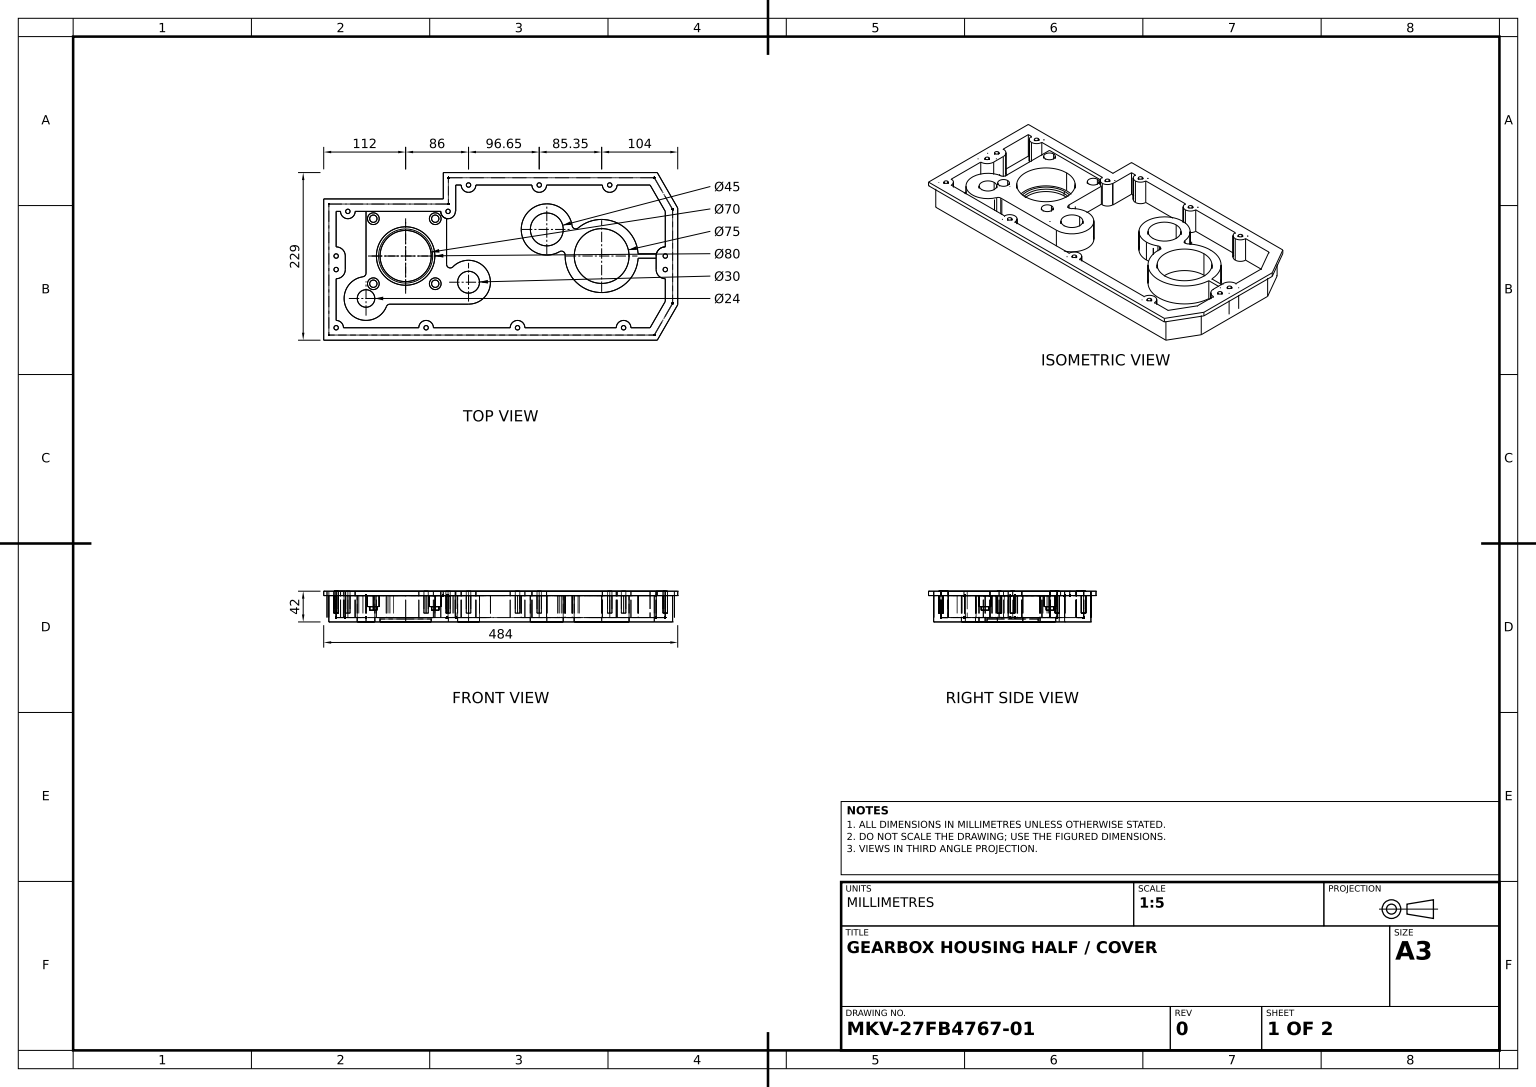
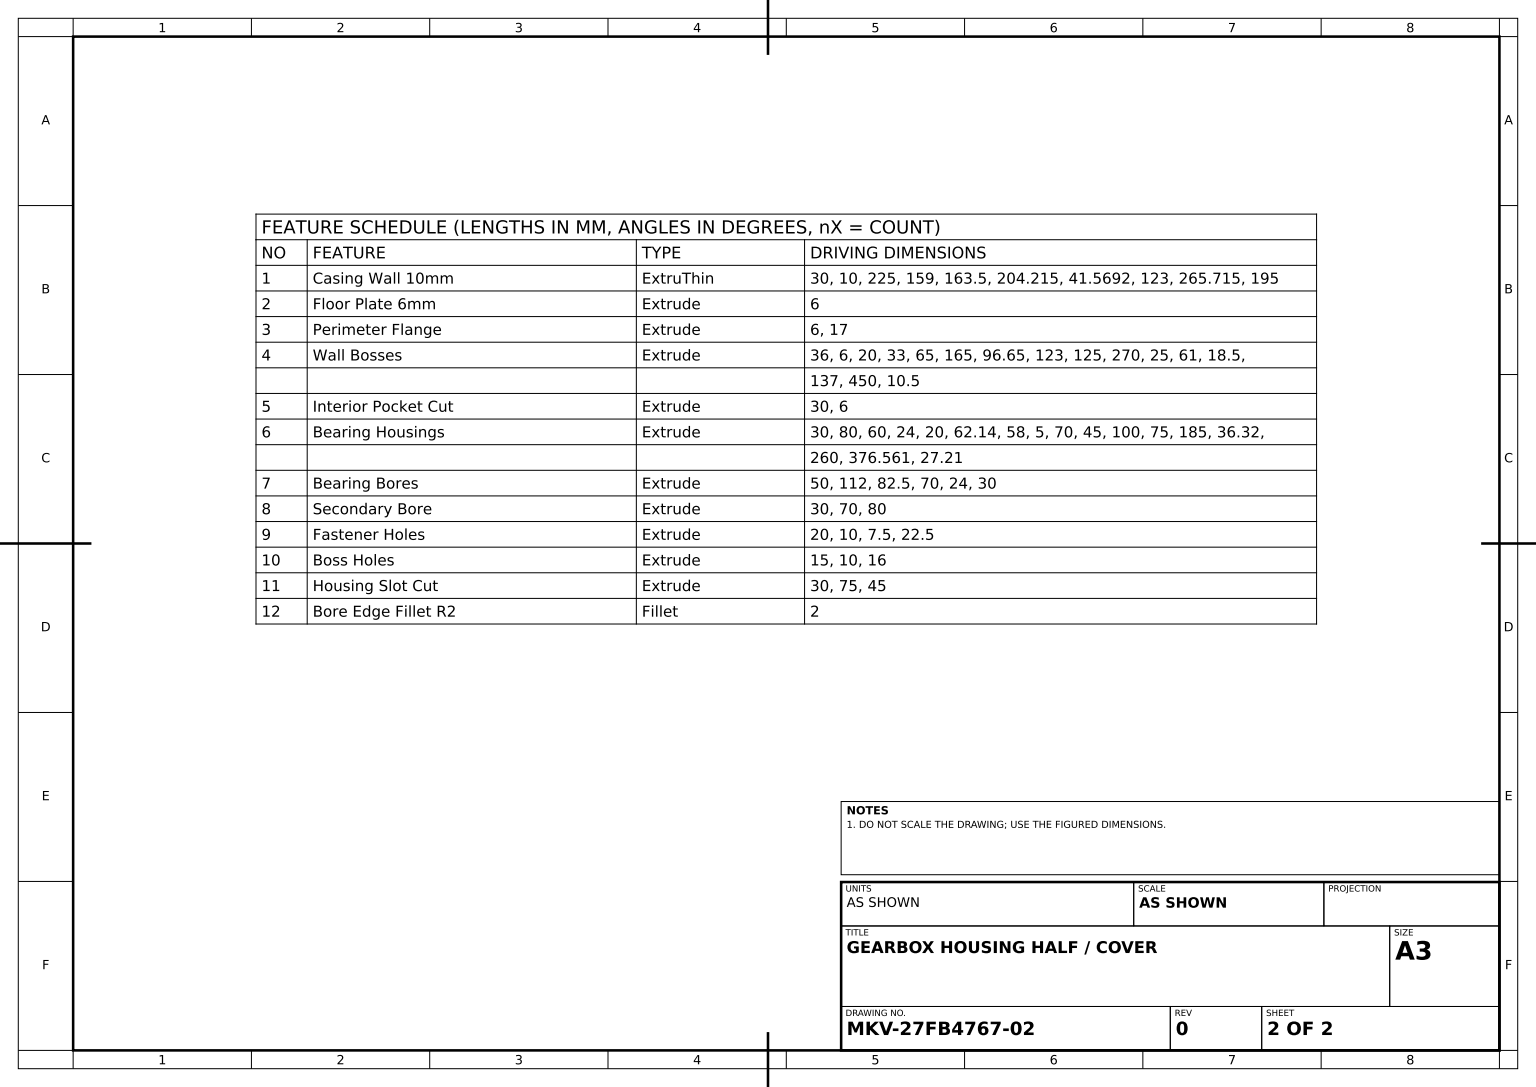
solid
v1 (225,36,-159)
v2 (204.21539,36,-195)
e1 v1 v2 LINE
v3 (204.21539,0,-195)
e2 v2 v3 LINE
v4 (225,0,-159)
e3 v4 v3 LINE
e4 v1 v4 LINE
face PLANE(AX(P(225,30,-159),D(-0.866025404,0,0.5),D(0.5,0,0.866025404))) [e1 e2 -e3 -e4]
v5 (-209,6,-162)
v6 (-209,36,-162)
e5 v5 v6 LINE
v7 (-209,6,-156)
e6 v7 v5 CIRCLE(AX(P(-209,6,-159),D(0,1,0),D(0,0,1)),3)
v8 (-209,36,-156)
e7 v7 v8 LINE
e8 v8 v6 CIRCLE(AX(P(-209,36,-159),D(0,1,0),D(0,0,1)),3)
face CYL(AX(P(-209,6,-159),D(0,1,0),D(0,0,1)),3) rev [-e5 -e6 e7 e8]
e9 v5 v7 CIRCLE(AX(P(-209,6,-159),D(0,1,0),D(0,0,1)),3)
face PLANE(AX(P(-209,6,-159),D(0,1,0),D(0,0,1))) [e9 e6]
v9 (-34,0,-195)
v10 (-34,36,-195)
e10 v9 v10 LINE
v11 (-44,36,-185)
e11 v11 v10 CIRCLE(AX(P(-44,36,-195),D(0,1,0),D(0,0,1)),10)
v12 (-44,0,-185)
e12 v12 v11 LINE
e13 v12 v9 CIRCLE(AX(P(-44,0,-195),D(0,1,0),D(0,0,1)),10)
face CYL(AX(P(-44,0,-195),D(0,1,0),D(0,0,1)),10) [e10 -e11 -e12 e13]
v13 (-89.5,30,-157)
v14 (-89.5,30,-141)
e14 v13 v14 CIRCLE(AX(P(-89.5,30,-149),D(0,1,0),D(0,0,1)),8)
v15 (-89.5,15,-141)
e15 v15 v14 LINE
v16 (-89.5,15,-157)
e16 v16 v15 CIRCLE(AX(P(-89.5,15,-149),D(0,1,0),D(0,0,1)),8)
e17 v16 v13 LINE
face CYL(AX(P(-89.5,15,-149),D(0,1,0),D(0,0,1)),8) rev [e14 -e15 -e16 e17]
v17 (242,36,-31.444864)
v18 (242,30,-31.444864)
e18 v17 v18 LINE
v19 (214.030345,36,17)
e19 v19 v17 LINE
v20 (214.030345,30,17)
e20 v19 v20 LINE
e21 v20 v18 LINE
face PLANE(AX(P(242,36,-31.444864),D(-0.866025404,0,-0.5),D(-0.5,0,0.866025404))) rev [-e18 -e19 e20 e21]
v21 (-44,30,-47.21)
v22 (-44,-6,-47.21)
e22 v21 v22 LINE
v23 (-44,-6,-77.21)
e23 v22 v23 CIRCLE(AX(P(-44,-6,-62.21),D(0,-1,0),D(0,0,-1)),15)
v24 (-44,30,-77.21)
e24 v24 v23 LINE
e25 v24 v21 CIRCLE(AX(P(-44,30,-62.21),D(0,1,0),D(0,0,1)),15)
face CYL(AX(P(-44,30,-62.21),D(0,-1,0),D(0,0,-1)),15) rev [e22 e23 -e24 e25]
v25 (159.030345,0,-195)
e26 v3 v25 LINE
v26 (159.030345,36,-195)
e27 v2 v26 LINE
e28 v25 v26 LINE
face PLANE(AX(P(-61.5,30,-195),D(0,0,1),D(1,0,0))) [-e26 -e2 e27 -e28]
v27 (-72,6,-162)
v28 (-72,36,-162)
e29 v27 v28 LINE
v29 (-72,36,-156)
e30 v28 v29 CIRCLE(AX(P(-72,36,-159),D(0,1,0),D(0,0,1)),3)
v30 (-72,6,-156)
e31 v30 v29 LINE
e32 v27 v30 CIRCLE(AX(P(-72,6,-159),D(0,1,0),D(0,0,1)),3)
face CYL(AX(P(-72,6,-159),D(0,1,0),D(0,0,1)),3) rev [e29 e30 -e31 -e32]
v31 (-215,0,0)
v32 (-215,36,0)
e33 v31 v32 LINE
v33 (-112,36,0)
e34 v32 v33 LINE
v34 (-112,0,0)
e35 v34 v33 LINE
e36 v31 v34 LINE
face PLANE(AX(P(-225,30,0),D(0,0,-1),D(-1,0,0))) [e33 e34 -e35 -e36]
v35 (139.030345,0,-195)
v36 (149.030345,0,-185)
e37 v35 v36 CIRCLE(AX(P(149.030345,0,-195),D(0,1,0),D(0,0,1)),10)
v37 (149.030345,36,-185)
e38 v36 v37 LINE
v38 (139.030345,36,-195)
e39 v38 v37 CIRCLE(AX(P(149.030345,36,-195),D(0,1,0),D(0,0,1)),10)
e40 v35 v38 LINE
face CYL(AX(P(149.030345,0,-195),D(0,1,0),D(0,0,1)),10) [e37 e38 -e39 -e40]
v39 (52.65,36,-192)
v40 (52.65,36,-198)
e41 v39 v40 CIRCLE(AX(P(52.65,36,-195),D(0,1,0),D(0,0,1)),3)
v41 (52.65,6,-198)
e42 v41 v40 LINE
v42 (52.65,6,-192)
e43 v42 v41 CIRCLE(AX(P(52.65,6,-195),D(0,1,0),D(0,0,1)),3)
e44 v42 v39 LINE
face CYL(AX(P(52.65,6,-195),D(0,1,0),D(0,0,1)),3) rev [e41 -e42 -e43 e44]
v43 (-225,0,-67)
v44 (-225,0,-10)
e45 v43 v44 LINE
v45 (-225,36,-67)
e46 v43 v45 LINE
v46 (-225,36,-10)
e47 v45 v46 LINE
e48 v44 v46 LINE
face PLANE(AX(P(-225,30,0),D(1,0,0),D(0,0,-1))) [-e45 e46 e47 -e48]
v47 (42.65,36,-195)
e49 v47 v10 LINE
v48 (42.65,0,-195)
e50 v48 v9 LINE
e51 v48 v47 LINE
face PLANE(AX(P(-61.5,30,-195),D(0,0,1),D(1,0,0))) [e49 -e10 -e50 e51]
v49 (63,30,-111.82)
v50 (63,-6,-111.82)
e52 v49 v50 LINE
v51 (63,30,-156.82)
e53 v49 v51 CIRCLE(AX(P(63,30,-134.32),D(0,1,0),D(0,0,1)),22.5)
v52 (63,-6,-156.82)
e54 v51 v52 LINE
e55 v52 v50 CIRCLE(AX(P(63,-6,-134.32),D(0,-1,0),D(0,0,-1)),22.5)
face CYL(AX(P(63,30,-134.32),D(0,-1,0),D(0,0,-1)),22.5) rev [-e52 e53 e54 e55]
e56 v30 v27 CIRCLE(AX(P(-72,6,-159),D(0,1,0),D(0,0,1)),3)
face PLANE(AX(P(-72,6,-159),D(0,1,0),D(0,0,1))) [e32 e56]
v53 (-102,36,-3)
v54 (-102,36,3)
e57 v53 v54 CIRCLE(AX(P(-102,36,0),D(0,1,0),D(0,0,1)),3)
v55 (-102,6,3)
e58 v55 v54 LINE
v56 (-102,6,-3)
e59 v56 v55 CIRCLE(AX(P(-102,6,0),D(0,1,0),D(0,0,1)),3)
e60 v56 v53 LINE
face CYL(AX(P(-102,6,0),D(0,1,0),D(0,0,1)),3) rev [e57 -e58 -e59 e60]
v57 (209.988893,30,10)
v58 (209.988893,-6,10)
e61 v57 v58 LINE
v59 (-235,30,10)
e62 v59 v57 LINE
v60 (-235,-6,10)
e63 v59 v60 LINE
e64 v58 v60 LINE
face PLANE(AX(P(0,30,10),D(0,0,-1),D(-1,0,0))) rev [-e61 -e62 e63 -e64]
v61 (225,6,-76.5)
v62 (225,6,-82.5)
e65 v61 v62 CIRCLE(AX(P(225,6,-79.5),D(0,1,0),D(0,0,1)),3)
v63 (225,36,-76.5)
e66 v61 v63 LINE
v64 (225,36,-82.5)
e67 v63 v64 CIRCLE(AX(P(225,36,-79.5),D(0,1,0),D(0,0,1)),3)
e68 v62 v64 LINE
face CYL(AX(P(225,6,-79.5),D(0,1,0),D(0,0,1)),3) rev [-e65 e66 e67 -e68]
v65 (80.522834,30,-104.022305)
v66 (80.522834,0,-104.022305)
e69 v65 v66 LINE
v67 (83.026096,0,-104.694063)
e70 v67 v66 CIRCLE(AX(P(83.026096,0,-99.694063),D(0,1,0),D(0,0,1)),5)
v68 (83.026096,30,-104.694063)
e71 v68 v67 LINE
e72 v68 v65 CIRCLE(AX(P(83.026096,30,-99.694063),D(0,1,0),D(0,0,1)),5)
face CYL(AX(P(83.026096,30,-99.694063),D(0,-1,0),D(0,0,-1)),5) rev [e69 -e70 -e71 e72]
v69 (-130,-6,-63)
v70 (-130,-6,-133)
e73 v69 v70 CIRCLE(AX(P(-130,-6,-98),D(0,-1,0),D(0,0,-1)),35)
e74 v70 v69 CIRCLE(AX(P(-130,-6,-98),D(0,-1,0),D(0,0,-1)),35)
v71 (235,-6,-33.320508)
e75 v71 v58 LINE
v72 (-235,-6,-169)
e76 v60 v72 LINE
v73 (-71.5,-6,-169)
e77 v72 v73 LINE
v74 (-71.5,-6,-205)
e78 v73 v74 LINE
v75 (209.988893,-6,-205)
e79 v74 v75 LINE
v76 (235,-6,-161.679492)
e80 v75 v76 LINE
e81 v76 v71 LINE
e82 v23 v22 CIRCLE(AX(P(-44,-6,-62.21),D(0,-1,0),D(0,0,-1)),15)
v77 (-184.14,-6,-28)
v78 (-184.14,-6,-52)
e83 v77 v78 CIRCLE(AX(P(-184.14,-6,-40),D(0,-1,0),D(0,0,-1)),12)
e84 v78 v77 CIRCLE(AX(P(-184.14,-6,-40),D(0,-1,0),D(0,0,-1)),12)
v79 (138,-6,-135.5)
v80 (138,-6,-60.5)
e85 v79 v80 CIRCLE(AX(P(138,-6,-98),D(0,-1,0),D(0,0,-1)),37.5)
e86 v80 v79 CIRCLE(AX(P(138,-6,-98),D(0,-1,0),D(0,0,-1)),37.5)
e87 v50 v52 CIRCLE(AX(P(63,-6,-134.32),D(0,-1,0),D(0,0,-1)),22.5)
face PLANE(AX(P(0,-6,0),D(0,-1,0),D(0,0,-1))) [-e73 -e74] [e75 e64 e76 e77 e78 e79 e80 e81] [-e23 -e82] [-e83 -e84] [-e85 -e86] [-e55 -e87]
v81 (187.909919,30,-101)
v82 (212.865339,30,-101)
e88 v81 v82 LINE
v83 (212.865339,0,-101)
e89 v82 v83 LINE
v84 (187.909919,0,-101)
e90 v84 v83 LINE
e91 v81 v84 LINE
face PLANE(AX(P(0,30,-101),D(0,0,-1),D(-1,0,0))) [e88 e89 -e90 -e91]
v85 (242,36,-163.555136)
v86 (242,30,-163.555136)
e92 v85 v86 LINE
e93 v17 v85 LINE
e94 v18 v86 LINE
face PLANE(AX(P(242,36,-163.555136),D(-1,0,0),D(0,0,1))) rev [-e92 -e93 e18 e94]
v87 (-62,0,-159)
v88 (-62,36,-159)
e95 v87 v88 LINE
v89 (-72,36,-149)
e96 v89 v88 CIRCLE(AX(P(-72,36,-159),D(0,1,0),D(0,0,1)),10)
v90 (-72,0,-149)
e97 v90 v89 LINE
e98 v90 v87 CIRCLE(AX(P(-72,0,-159),D(0,1,0),D(0,0,1)),10)
face CYL(AX(P(-72,0,-159),D(0,1,0),D(0,0,1)),10) [e95 -e96 -e97 e98]
v91 (-225,36,-101)
v92 (-225,36,-95)
e99 v91 v92 CIRCLE(AX(P(-225,36,-98),D(0,1,0),D(0,0,1)),3)
v93 (-225,6,-95)
e100 v93 v92 LINE
v94 (-225,6,-101)
e101 v94 v93 CIRCLE(AX(P(-225,6,-98),D(0,1,0),D(0,0,1)),3)
e102 v94 v91 LINE
face CYL(AX(P(-225,6,-98),D(0,1,0),D(0,0,1)),3) rev [e99 -e100 -e101 e102]
v95 (-209,0,-149)
v96 (-209,36,-149)
e103 v95 v96 LINE
v97 (-219,36,-159)
e104 v97 v96 CIRCLE(AX(P(-209,36,-159),D(0,1,0),D(0,0,1)),10)
v98 (-219,0,-159)
e105 v98 v97 LINE
e106 v98 v95 CIRCLE(AX(P(-209,0,-159),D(0,1,0),D(0,0,1)),10)
face CYL(AX(P(-209,0,-159),D(0,1,0),D(0,0,1)),10) [e103 -e104 -e105 e106]
v99 (23,6,-3)
v100 (23,36,-3)
e107 v99 v100 LINE
v101 (23,36,3)
e108 v100 v101 CIRCLE(AX(P(23,36,0),D(0,1,0),D(0,0,1)),3)
v102 (23,6,3)
e109 v102 v101 LINE
e110 v99 v102 CIRCLE(AX(P(23,6,0),D(0,1,0),D(0,0,1)),3)
face CYL(AX(P(23,6,0),D(0,1,0),D(0,0,1)),3) rev [e107 e108 -e109 -e110]
v103 (-174.14,10,-144)
v104 (-174.14,15,-144)
e111 v103 v104 LINE
v105 (-174.14,10,-154)
e112 v105 v103 CIRCLE(AX(P(-174.14,10,-149),D(0,1,0),D(0,0,1)),5)
v106 (-174.14,15,-154)
e113 v105 v106 LINE
e114 v106 v104 CIRCLE(AX(P(-174.14,15,-149),D(0,1,0),D(0,0,1)),5)
face CYL(AX(P(-174.14,10,-149),D(0,1,0),D(0,0,1)),5) rev [-e111 -e112 e113 e114]
v107 (-225,36,-3)
v108 (-225,36,3)
e115 v107 v108 CIRCLE(AX(P(-225,36,0),D(0,1,0),D(0,0,1)),3)
v109 (-225,6,3)
e116 v109 v108 LINE
v110 (-225,6,-3)
e117 v110 v109 CIRCLE(AX(P(-225,6,0),D(0,1,0),D(0,0,1)),3)
e118 v110 v107 LINE
face CYL(AX(P(-225,6,0),D(0,1,0),D(0,0,1)),3) rev [e115 -e116 -e117 e118]
v111 (-156.214818,30,-29.037143)
v112 (-156.214818,0,-29.037143)
e119 v111 v112 LINE
v113 (-188.425714,30,-69.6923)
e120 v113 v111 CIRCLE(AX(P(-184.14,30,-40),D(0,1,0),D(0,0,1)),30)
v114 (-188.425714,0,-69.6923)
e121 v113 v114 LINE
e122 v114 v112 CIRCLE(AX(P(-184.14,0,-40),D(0,1,0),D(0,0,1)),30)
face CYL(AX(P(-184.14,30,-40),D(0,-1,0),D(0,0,-1)),30) [-e119 -e120 e121 e122]
v115 (-130,0,-58)
v116 (-130,0,-138)
e123 v115 v116 CIRCLE(AX(P(-130,0,-98),D(0,1,0),D(0,0,1)),40)
e124 v116 v115 CIRCLE(AX(P(-130,0,-98),D(0,1,0),D(0,0,1)),40)
v117 (-130,0,-61)
v118 (-130,0,-135)
e125 v117 v118 CIRCLE(AX(P(-130,0,-98),D(0,-1,0),D(0,0,1)),37)
e126 v118 v117 CIRCLE(AX(P(-130,0,-98),D(0,-1,0),D(0,0,1)),37)
face PLANE(AX(P(-130,0,-98),D(0,1,0),D(0,0,1))) [e123 e124] [e125 e126]
v119 (88.023723,30,-99.540058)
v120 (187.909919,30,-95)
e127 v119 v120 CIRCLE(AX(P(138,30,-98),D(0,1,0),D(0,0,1)),50)
v121 (88.023723,0,-99.540058)
e128 v119 v121 LINE
v122 (187.909919,0,-95)
e129 v121 v122 CIRCLE(AX(P(138,0,-98),D(0,1,0),D(0,0,1)),50)
e130 v120 v122 LINE
face CYL(AX(P(138,30,-98),D(0,-1,0),D(0,0,-1)),50) [-e127 e128 e129 -e130]
v123 (-89.5,15,-68.155644)
v124 (-89.5,15,-52.155644)
e131 v123 v124 CIRCLE(AX(P(-89.5,15,-60.155644),D(0,1,0),D(0,0,1)),8)
e132 v124 v123 CIRCLE(AX(P(-89.5,15,-60.155644),D(0,1,0),D(0,0,1)),8)
v125 (-89.5,15,-55.155644)
v126 (-89.5,15,-65.155644)
e133 v125 v126 CIRCLE(AX(P(-89.5,15,-60.155644),D(0,1,0),D(0,0,1)),5)
e134 v126 v125 CIRCLE(AX(P(-89.5,15,-60.155644),D(0,1,0),D(0,0,1)),5)
face PLANE(AX(P(-89.5,15,-60.155644),D(0,1,0),D(0,0,1))) [e131 e132] [-e133 -e134]
v127 (225,6,-101)
v128 (225,36,-101)
e135 v127 v128 LINE
v129 (225,6,-95)
e136 v129 v127 CIRCLE(AX(P(225,6,-98),D(0,1,0),D(0,0,1)),3)
v130 (225,36,-95)
e137 v129 v130 LINE
e138 v130 v128 CIRCLE(AX(P(225,36,-98),D(0,1,0),D(0,0,1)),3)
face CYL(AX(P(225,6,-98),D(0,1,0),D(0,0,1)),3) rev [-e135 -e136 e137 e138]
v131 (212.5,30,-98)
v132 (212.5,36,-98)
e139 v131 v132 LINE
v133 (212.5,30,-95)
e140 v133 v131 LINE
v134 (212.5,0,-95)
e141 v133 v134 LINE
v135 (212.5,0,-79.5)
e142 v134 v135 LINE
v136 (212.5,36,-79.5)
e143 v135 v136 LINE
e144 v132 v136 LINE
face PLANE(AX(P(212.5,0,0),D(-1,0,0),D(0,0,1))) [-e139 -e140 e141 e142 e143 -e144]
v137 (-225,36,-159)
e145 v97 v137 LINE
v138 (-225,0,-159)
e146 v137 v138 LINE
e147 v98 v138 LINE
face PLANE(AX(P(-225,30,-159),D(0,0,1),D(1,0,0))) [e105 e145 e146 -e147]
v139 (-225,6,-82.5)
v140 (-225,36,-82.5)
e148 v139 v140 LINE
v141 (-225,6,-76.5)
e149 v141 v139 CIRCLE(AX(P(-225,6,-79.5),D(0,1,0),D(0,0,1)),3)
v142 (-225,36,-76.5)
e150 v141 v142 LINE
e151 v142 v140 CIRCLE(AX(P(-225,36,-79.5),D(0,1,0),D(0,0,1)),3)
face CYL(AX(P(-225,6,-79.5),D(0,1,0),D(0,0,1)),3) rev [-e148 -e149 e150 e151]
v143 (-89.5,15,-154)
v144 (-89.5,15,-144)
e152 v143 v144 CIRCLE(AX(P(-89.5,15,-149),D(0,1,0),D(0,0,1)),5)
v145 (-89.5,10,-144)
e153 v145 v144 LINE
v146 (-89.5,10,-154)
e154 v146 v145 CIRCLE(AX(P(-89.5,10,-149),D(0,1,0),D(0,0,1)),5)
e155 v146 v143 LINE
face CYL(AX(P(-89.5,10,-149),D(0,1,0),D(0,0,1)),5) rev [e152 -e153 -e154 e155]
v147 (-44,30,-32.21)
v148 (-151.560622,30,-32.21)
e156 v147 v148 LINE
v149 (-151.560622,0,-32.21)
e157 v148 v149 LINE
v150 (-44,0,-32.21)
e158 v150 v149 LINE
e159 v147 v150 LINE
face PLANE(AX(P(0,30,-32.21),D(0,0,1),D(1,0,0))) [e156 e157 -e158 -e159]
v151 (-89.5,30,-68.155644)
e160 v123 v151 LINE
v152 (-89.5,30,-52.155644)
e161 v151 v152 CIRCLE(AX(P(-89.5,30,-60.155644),D(0,1,0),D(0,0,1)),8)
e162 v124 v152 LINE
face CYL(AX(P(-89.5,15,-60.155644),D(0,1,0),D(0,0,1)),8) rev [e160 e161 -e162 -e131]
v153 (62.65,36,-195)
e163 v38 v153 LINE
v154 (62.65,0,-195)
e164 v154 v153 LINE
e165 v35 v154 LINE
face PLANE(AX(P(-61.5,30,-195),D(0,0,1),D(1,0,0))) [e40 e163 -e164 -e165]
v155 (-74,30,-86.704897)
v156 (-74,0,-86.704897)
e166 v155 v156 LINE
v157 (-65.428571,30,-83.205626)
e167 v155 v157 CIRCLE(AX(P(-69,30,-86.704897),D(0,1,0),D(0,0,1)),5)
v158 (-65.428571,0,-83.205626)
e168 v157 v158 LINE
e169 v156 v158 CIRCLE(AX(P(-69,0,-86.704897),D(0,1,0),D(0,0,1)),5)
face CYL(AX(P(-69,30,-86.704897),D(0,-1,0),D(0,0,-1)),5) rev [-e166 e167 e168 -e169]
v159 (-44,30,-92.21)
v160 (-44,0,-92.21)
e170 v159 v160 LINE
e171 v160 v158 CIRCLE(AX(P(-44,0,-62.21),D(0,1,0),D(0,0,1)),30)
e172 v159 v157 CIRCLE(AX(P(-44,30,-62.21),D(0,1,0),D(0,0,1)),30)
face CYL(AX(P(-44,30,-62.21),D(0,-1,0),D(0,0,-1)),30) [e170 e171 -e168 -e172]
v161 (168,6,-3)
v162 (168,36,-3)
e173 v161 v162 LINE
v163 (168,36,3)
e174 v162 v163 CIRCLE(AX(P(168,36,0),D(0,1,0),D(0,0,1)),3)
v164 (168,6,3)
e175 v164 v163 LINE
e176 v161 v164 CIRCLE(AX(P(168,6,0),D(0,1,0),D(0,0,1)),3)
face CYL(AX(P(168,6,0),D(0,1,0),D(0,0,1)),3) rev [e173 e174 -e175 -e176]
v165 (138,30,-148)
e177 v81 v165 CIRCLE(AX(P(138,30,-98),D(0,1,0),D(0,0,1)),50)
v166 (138,0,-148)
e178 v84 v166 CIRCLE(AX(P(138,0,-98),D(0,1,0),D(0,0,1)),50)
e179 v165 v166 LINE
face CYL(AX(P(138,30,-98),D(0,-1,0),D(0,0,-1)),50) [-e177 e91 e178 -e179]
v167 (-89.5,10,-55.155644)
e180 v167 v125 LINE
v168 (-89.5,10,-65.155644)
e181 v168 v167 CIRCLE(AX(P(-89.5,10,-60.155644),D(0,1,0),D(0,0,1)),5)
e182 v168 v126 LINE
face CYL(AX(P(-89.5,10,-60.155644),D(0,1,0),D(0,0,1)),5) rev [e134 -e180 -e181 e182]
v169 (-44,36,-192)
v170 (-44,36,-198)
e183 v169 v170 CIRCLE(AX(P(-44,36,-195),D(0,1,0),D(0,0,1)),3)
v171 (-44,6,-198)
e184 v171 v170 LINE
v172 (-44,6,-192)
e185 v172 v171 CIRCLE(AX(P(-44,6,-195),D(0,1,0),D(0,0,1)),3)
e186 v172 v169 LINE
face CYL(AX(P(-44,6,-195),D(0,1,0),D(0,0,1)),3) rev [e183 -e184 -e185 e186]
v173 (-92,36,0)
e187 v173 v33 CIRCLE(AX(P(-102,36,0),D(0,1,0),D(0,0,1)),10)
v174 (-92,0,0)
e188 v174 v173 LINE
e189 v174 v34 CIRCLE(AX(P(-102,0,0),D(0,1,0),D(0,0,1)),10)
face CYL(AX(P(-102,0,0),D(0,1,0),D(0,0,1)),10) [-e187 -e188 e189 e35]
v175 (-235,30,-169)
e190 v175 v59 LINE
e191 v175 v72 LINE
face PLANE(AX(P(-235,30,0),D(1,0,0),D(0,0,-1))) rev [-e76 -e63 -e190 e191]
v176 (-212.5,36,-98)
v177 (-225,36,-110.5)
e192 v176 v177 CIRCLE(AX(P(-225,36,-98),D(0,1,0),D(0,0,1)),12.5)
v178 (-212.5,0,-98)
e193 v178 v176 LINE
v179 (-225,0,-110.5)
e194 v178 v179 CIRCLE(AX(P(-225,0,-98),D(0,1,0),D(0,0,1)),12.5)
e195 v179 v177 LINE
face CYL(AX(P(-225,0,-98),D(0,1,0),D(0,0,1)),12.5) [-e192 -e193 e194 e195]
v180 (-74,0,-149.202041)
e196 v180 v90 CIRCLE(AX(P(-72,0,-159),D(0,1,0),D(0,0,1)),10)
v181 (-82,36,-159)
e197 v181 v89 CIRCLE(AX(P(-72,36,-159),D(0,1,0),D(0,0,1)),10)
v182 (-82,30,-159)
e198 v182 v181 LINE
v183 (-74,30,-149.202041)
e199 v183 v182 CIRCLE(AX(P(-72,30,-159),D(0,-1,0),D(0,0,1)),10)
e200 v183 v180 LINE
face CYL(AX(P(-72,0,-159),D(0,1,0),D(0,0,1)),10) [e196 e97 -e197 -e198 -e199 e200]
e201 v122 v134 LINE
e202 v120 v133 LINE
face PLANE(AX(P(0,30,-95),D(0,0,-1),D(-1,0,0))) rev [e130 e201 -e141 -e202]
v184 (105.802941,30,-136.25375)
e203 v165 v184 CIRCLE(AX(P(138,30,-98),D(0,1,0),D(0,0,1)),50)
v185 (105.802941,0,-136.25375)
e204 v166 v185 CIRCLE(AX(P(138,0,-98),D(0,1,0),D(0,0,1)),50)
e205 v184 v185 LINE
face CYL(AX(P(138,30,-98),D(0,-1,0),D(0,0,-1)),50) [-e203 e179 e204 -e205]
v186 (149.030345,6,-198)
v187 (149.030345,36,-198)
e206 v186 v187 LINE
v188 (149.030345,6,-192)
e207 v188 v186 CIRCLE(AX(P(149.030345,6,-195),D(0,1,0),D(0,0,1)),3)
v189 (149.030345,36,-192)
e208 v188 v189 LINE
e209 v189 v187 CIRCLE(AX(P(149.030345,36,-195),D(0,1,0),D(0,0,1)),3)
face CYL(AX(P(149.030345,6,-195),D(0,1,0),D(0,0,1)),3) rev [-e206 -e207 e208 e209]
v190 (-242,36,17)
e210 v190 v19 LINE
v191 (-242,30,17)
e211 v190 v191 LINE
e212 v191 v20 LINE
face PLANE(AX(P(214.030345,36,17),D(0,0,-1),D(-1,0,0))) rev [-e210 e211 e212 -e20]
e213 v31 v44 CIRCLE(AX(P(-225,0,0),D(0,1,0),D(0,0,1)),10)
e214 v32 v46 CIRCLE(AX(P(-225,36,0),D(0,1,0),D(0,0,1)),10)
face CYL(AX(P(-225,0,0),D(0,1,0),D(0,0,1)),10) [-e33 e213 e48 -e214]
v192 (225,36,-110.5)
e215 v192 v1 LINE
v193 (225,0,-110.5)
e216 v193 v4 LINE
e217 v193 v192 LINE
face PLANE(AX(P(225,30,-159),D(-1,0,0),D(0,0,1))) [e215 e4 -e216 e217]
v194 (-242,36,-176)
e218 v194 v190 LINE
v195 (-242,30,-176)
e219 v194 v195 LINE
e220 v195 v191 LINE
face PLANE(AX(P(-242,36,17),D(1,0,0),D(0,0,-1))) rev [-e218 e219 e220 -e211]
e221 v187 v189 CIRCLE(AX(P(149.030345,36,-195),D(0,1,0),D(0,0,1)),3)
e222 v186 v188 CIRCLE(AX(P(149.030345,6,-195),D(0,1,0),D(0,0,1)),3)
face CYL(AX(P(149.030345,6,-195),D(0,1,0),D(0,0,1)),3) rev [e206 e221 -e208 -e222]
e223 v14 v13 CIRCLE(AX(P(-89.5,30,-149),D(0,1,0),D(0,0,1)),8)
v196 (-184.14,30,-159)
e224 v182 v196 LINE
v197 (-184.14,30,-74.641016)
e225 v197 v196 LINE
e226 v197 v113 CIRCLE(AX(P(-189.14,30,-74.641016),D(0,-1,0),D(0,0,1)),5)
e227 v148 v111 CIRCLE(AX(P(-151.560622,30,-27.21),D(0,1,0),D(0,0,1)),5)
e228 v147 v159 CIRCLE(AX(P(-44,30,-62.21),D(0,1,0),D(0,0,1)),30)
e229 v155 v183 LINE
e230 v21 v24 CIRCLE(AX(P(-44,30,-62.21),D(0,1,0),D(0,0,1)),15)
v198 (-174.14,30,-52.155644)
v199 (-174.14,30,-68.155644)
e231 v198 v199 CIRCLE(AX(P(-174.14,30,-60.155644),D(0,1,0),D(0,0,1)),8)
e232 v199 v198 CIRCLE(AX(P(-174.14,30,-60.155644),D(0,1,0),D(0,0,1)),8)
v200 (-174.14,30,-157)
v201 (-174.14,30,-141)
e233 v200 v201 CIRCLE(AX(P(-174.14,30,-149),D(0,1,0),D(0,0,1)),8)
e234 v201 v200 CIRCLE(AX(P(-174.14,30,-149),D(0,1,0),D(0,0,1)),8)
e235 v152 v151 CIRCLE(AX(P(-89.5,30,-60.155644),D(0,1,0),D(0,0,1)),8)
v202 (-184.14,30,-28)
v203 (-184.14,30,-52)
e236 v202 v203 CIRCLE(AX(P(-184.14,30,-40),D(0,1,0),D(0,0,1)),12)
e237 v203 v202 CIRCLE(AX(P(-184.14,30,-40),D(0,1,0),D(0,0,1)),12)
v204 (-130,30,-138)
v205 (-130,30,-58)
e238 v204 v205 CIRCLE(AX(P(-130,30,-98),D(0,1,0),D(0,0,1)),40)
e239 v205 v204 CIRCLE(AX(P(-130,30,-98),D(0,1,0),D(0,0,1)),40)
face PLANE(AX(P(0,30,0),D(0,1,0),D(0,0,1))) [-e14 -e223] [e224 -e225 e226 e120 -e227 -e156 e228 e172 -e167 e229 e199] [-e25 -e230] [-e231 -e232] [-e233 -e234] [-e161 -e235] [-e236 -e237] [-e238 -e239]
v206 (214.030345,36,-212)
v207 (-78.5,36,-212)
e240 v206 v207 LINE
v208 (214.030345,30,-212)
e241 v206 v208 LINE
v209 (-78.5,30,-212)
e242 v208 v209 LINE
e243 v207 v209 LINE
face PLANE(AX(P(-78.5,36,-212),D(0,0,1),D(1,0,0))) rev [-e240 e241 e242 -e243]
e244 v109 v110 CIRCLE(AX(P(-225,6,0),D(0,1,0),D(0,0,1)),3)
e245 v108 v107 CIRCLE(AX(P(-225,36,0),D(0,1,0),D(0,0,1)),3)
face CYL(AX(P(-225,6,0),D(0,1,0),D(0,0,1)),3) rev [-e118 -e244 e116 e245]
e246 v137 v177 LINE
e247 v138 v179 LINE
face PLANE(AX(P(-225,30,0),D(1,0,0),D(0,0,-1))) [e246 -e195 -e247 -e146]
e248 v127 v129 CIRCLE(AX(P(225,6,-98),D(0,1,0),D(0,0,1)),3)
e249 v128 v130 CIRCLE(AX(P(225,36,-98),D(0,1,0),D(0,0,1)),3)
face CYL(AX(P(225,6,-98),D(0,1,0),D(0,0,1)),3) rev [-e248 e135 e249 -e137]
e250 v163 v162 CIRCLE(AX(P(168,36,0),D(0,1,0),D(0,0,1)),3)
e251 v164 v161 CIRCLE(AX(P(168,6,0),D(0,1,0),D(0,0,1)),3)
face CYL(AX(P(168,6,0),D(0,1,0),D(0,0,1)),3) rev [e175 e250 -e173 -e251]
e252 v167 v168 CIRCLE(AX(P(-89.5,10,-60.155644),D(0,1,0),D(0,0,1)),5)
face PLANE(AX(P(-89.5,10,-60.155644),D(0,1,0),D(0,0,1))) [e181 e252]
v210 (-54,0,-195)
e253 v210 v12 CIRCLE(AX(P(-44,0,-195),D(0,1,0),D(0,0,1)),10)
v211 (-61.5,0,-195)
e254 v210 v211 LINE
v212 (-61.5,0,-159)
e255 v211 v212 LINE
e256 v212 v87 LINE
e257 v156 v180 LINE
e258 v150 v160 CIRCLE(AX(P(-44,0,-62.21),D(0,1,0),D(0,0,1)),30)
e259 v149 v112 CIRCLE(AX(P(-151.560622,0,-27.21),D(0,1,0),D(0,0,1)),5)
v213 (-184.14,0,-74.641016)
e260 v213 v114 CIRCLE(AX(P(-189.14,0,-74.641016),D(0,-1,0),D(0,0,1)),5)
v214 (-184.14,0,-159)
e261 v213 v214 LINE
v215 (-199,0,-159)
e262 v214 v215 LINE
e263 v95 v215 CIRCLE(AX(P(-209,0,-159),D(0,1,0),D(0,0,1)),10)
v216 (-212.5,0,-79.5)
e264 v178 v216 LINE
e265 v43 v216 CIRCLE(AX(P(-225,0,-79.5),D(0,1,0),D(0,0,1)),12.5)
v217 (13,0,0)
e266 v174 v217 LINE
v218 (33,0,0)
e267 v218 v217 CIRCLE(AX(P(23,0,0),D(0,1,0),D(0,0,1)),10)
v219 (158,0,0)
e268 v218 v219 LINE
v220 (178,0,0)
e269 v220 v219 CIRCLE(AX(P(168,0,0),D(0,1,0),D(0,0,1)),10)
v221 (204.21539,0,0)
e270 v220 v221 LINE
v222 (225,0,-36)
e271 v221 v222 LINE
v223 (225,0,-67)
e272 v222 v223 LINE
e273 v135 v223 CIRCLE(AX(P(225,0,-79.5),D(0,1,0),D(0,0,1)),12.5)
e274 v121 v67 CIRCLE(AX(P(83.026096,0,-99.694063),D(0,1,0),D(0,0,1)),5)
v224 (63,0,-99.32)
e275 v224 v66 CIRCLE(AX(P(63,0,-134.32),D(0,1,0),D(0,0,1)),35)
v225 (63,0,-169.32)
e276 v225 v224 CIRCLE(AX(P(63,0,-134.32),D(0,1,0),D(0,0,1)),35)
v226 (97.63533,0,-139.359234)
e277 v226 v225 CIRCLE(AX(P(63,0,-134.32),D(0,1,0),D(0,0,1)),35)
e278 v185 v226 CIRCLE(AX(P(102.583235,0,-140.079125),D(0,-1,0),D(0,0,1)),5)
e279 v193 v83 CIRCLE(AX(P(225,0,-98),D(0,1,0),D(0,0,1)),12.5)
e280 v36 v25 CIRCLE(AX(P(149.030345,0,-195),D(0,1,0),D(0,0,1)),10)
v227 (52.65,0,-185)
e281 v227 v154 CIRCLE(AX(P(52.65,0,-195),D(0,1,0),D(0,0,1)),10)
e282 v48 v227 CIRCLE(AX(P(52.65,0,-195),D(0,1,0),D(0,0,1)),10)
face PLANE(AX(P(0,0,0),D(0,-1,0),D(0,0,-1))) rev [-e13 -e253 e254 e255 e256 -e98 -e196 -e257 e169 -e171 -e258 e158 e259 -e122 -e260 e261 e262 -e263 -e106 e147 e247 -e194 e264 -e265 e45 -e213 e36 -e189 e266 -e267 e268 -e269 e270 e271 e272 -e273 -e142 -e201 -e129 e274 e70 -e275 -e276 -e277 -e278 -e204 -e178 e90 -e279 e216 e3 e26 -e280 -e37 e165 -e281 -e282 e50]
face PLANE(AX(P(149.030345,6,-195),D(0,1,0),D(0,0,1))) [e207 e222]
v228 (52.65,36,-185)
e283 v228 v153 CIRCLE(AX(P(52.65,36,-195),D(0,1,0),D(0,0,1)),10)
e284 v227 v228 LINE
face CYL(AX(P(52.65,0,-195),D(0,1,0),D(0,0,1)),10) [-e283 -e284 e281 e164]
e285 v55 v56 CIRCLE(AX(P(-102,6,0),D(0,1,0),D(0,0,1)),3)
e286 v54 v53 CIRCLE(AX(P(-102,36,0),D(0,1,0),D(0,0,1)),3)
face CYL(AX(P(-102,6,0),D(0,1,0),D(0,0,1)),3) rev [-e285 e58 e286 -e60]
v229 (178,36,0)
e287 v220 v229 LINE
v230 (158,36,0)
e288 v219 v230 LINE
e289 v229 v230 CIRCLE(AX(P(168,36,0),D(0,1,0),D(0,0,1)),10)
face CYL(AX(P(168,0,0),D(0,1,0),D(0,0,1)),10) [-e287 e269 e288 -e289]
v231 (-54,36,-195)
e290 v210 v231 LINE
e291 v231 v11 CIRCLE(AX(P(-44,36,-195),D(0,1,0),D(0,0,1)),10)
face CYL(AX(P(-44,0,-195),D(0,1,0),D(0,0,1)),10) [-e290 e253 e12 -e291]
v232 (-174.14,10,-55.155644)
v233 (-174.14,10,-65.155644)
e292 v232 v233 CIRCLE(AX(P(-174.14,10,-60.155644),D(0,1,0),D(0,0,1)),5)
e293 v233 v232 CIRCLE(AX(P(-174.14,10,-60.155644),D(0,1,0),D(0,0,1)),5)
face PLANE(AX(P(-174.14,10,-60.155644),D(0,1,0),D(0,0,1))) [e292 e293]
v234 (138,30,-135.5)
e294 v234 v79 LINE
v235 (138,30,-60.5)
e295 v234 v235 CIRCLE(AX(P(138,30,-98),D(0,1,0),D(0,0,1)),37.5)
e296 v235 v80 LINE
face CYL(AX(P(138,30,-98),D(0,-1,0),D(0,0,-1)),37.5) rev [-e294 e295 e296 e86]
v236 (-212.5,36,-79.5)
e297 v216 v236 LINE
e298 v45 v236 CIRCLE(AX(P(-225,36,-79.5),D(0,1,0),D(0,0,1)),12.5)
face CYL(AX(P(-225,0,-79.5),D(0,1,0),D(0,0,1)),12.5) [e265 e297 -e298 -e46]
face CYL(AX(P(-89.5,10,-60.155644),D(0,1,0),D(0,0,1)),5) rev [e180 e133 -e182 -e252]
v237 (-174.14,15,-68.155644)
e299 v237 v199 LINE
v238 (-174.14,15,-52.155644)
e300 v238 v237 CIRCLE(AX(P(-174.14,15,-60.155644),D(0,1,0),D(0,0,1)),8)
e301 v238 v198 LINE
face CYL(AX(P(-174.14,15,-60.155644),D(0,1,0),D(0,0,1)),8) rev [e231 -e299 -e300 e301]
v239 (235,30,-33.320508)
v240 (235,30,-161.679492)
e302 v239 v240 LINE
e303 v239 v71 LINE
e304 v240 v76 LINE
face PLANE(AX(P(235,30,0),D(-1,0,0),D(0,0,1))) rev [-e302 e303 -e81 -e304]
e305 v41 v42 CIRCLE(AX(P(52.65,6,-195),D(0,1,0),D(0,0,1)),3)
e306 v40 v39 CIRCLE(AX(P(52.65,36,-195),D(0,1,0),D(0,0,1)),3)
face CYL(AX(P(52.65,6,-195),D(0,1,0),D(0,0,1)),3) rev [-e44 -e305 e42 e306]
e307 v139 v141 CIRCLE(AX(P(-225,6,-79.5),D(0,1,0),D(0,0,1)),3)
face PLANE(AX(P(-225,6,-79.5),D(0,1,0),D(0,0,1))) [e149 e307]
face PLANE(AX(P(-102,6,0),D(0,1,0),D(0,0,1))) [e285 e59]
v241 (63,30,-99.32)
e308 v241 v224 LINE
v242 (63,30,-169.32)
e309 v242 v241 CIRCLE(AX(P(63,30,-134.32),D(0,1,0),D(0,0,1)),35)
e310 v242 v225 LINE
face CYL(AX(P(63,30,-134.32),D(0,-1,0),D(0,0,-1)),35) [-e308 -e309 e310 e276]
e311 v6 v8 CIRCLE(AX(P(-209,36,-159),D(0,1,0),D(0,0,1)),3)
v243 (-78.5,36,-176)
e312 v207 v243 LINE
e313 v243 v194 LINE
e314 v85 v206 LINE
e315 v192 v132 CIRCLE(AX(P(225,36,-98),D(0,1,0),D(0,0,1)),12.5)
v244 (225,36,-67)
e316 v136 v244 CIRCLE(AX(P(225,36,-79.5),D(0,1,0),D(0,0,1)),12.5)
v245 (225,36,-36)
e317 v245 v244 LINE
v246 (204.21539,36,0)
e318 v246 v245 LINE
e319 v229 v246 LINE
v247 (33,36,0)
e320 v247 v230 LINE
v248 (13,36,0)
e321 v247 v248 CIRCLE(AX(P(23,36,0),D(0,1,0),D(0,0,1)),10)
e322 v173 v248 LINE
e323 v176 v236 LINE
v249 (-199,36,-159)
e324 v96 v249 CIRCLE(AX(P(-209,36,-159),D(0,1,0),D(0,0,1)),10)
e325 v181 v249 LINE
v250 (-61.5,36,-159)
e326 v250 v88 LINE
v251 (-61.5,36,-195)
e327 v251 v250 LINE
e328 v231 v251 LINE
e329 v47 v228 CIRCLE(AX(P(52.65,36,-195),D(0,1,0),D(0,0,1)),10)
e330 v37 v26 CIRCLE(AX(P(149.030345,36,-195),D(0,1,0),D(0,0,1)),10)
e331 v64 v63 CIRCLE(AX(P(225,36,-79.5),D(0,1,0),D(0,0,1)),3)
e332 v92 v91 CIRCLE(AX(P(-225,36,-98),D(0,1,0),D(0,0,1)),3)
e333 v101 v100 CIRCLE(AX(P(23,36,0),D(0,1,0),D(0,0,1)),3)
e334 v170 v169 CIRCLE(AX(P(-44,36,-195),D(0,1,0),D(0,0,1)),3)
e335 v29 v28 CIRCLE(AX(P(-72,36,-159),D(0,1,0),D(0,0,1)),3)
e336 v140 v142 CIRCLE(AX(P(-225,36,-79.5),D(0,1,0),D(0,0,1)),3)
face PLANE(AX(P(0,36,0),D(0,-1,0),D(0,0,-1))) rev [-e174 -e250] [-e311 -e8] [e240 e312 e313 e218 e210 e19 e93 e314] [-e41 -e306] [-e57 -e286] [-e115 -e245] [-e209 -e221] [-e27 -e1 -e215 e315 e144 e316 -e317 -e318 -e319 e289 -e320 e321 -e322 e187 -e34 e214 -e47 e298 -e323 e192 -e246 -e145 e104 e324 -e325 e197 e96 -e326 -e327 -e328 e291 e11 -e49 e329 e283 -e163 e39 e330] [-e67 -e331] [-e249 -e138] [-e99 -e332] [-e333 -e108] [-e183 -e334] [-e335 -e30] [-e336 -e151]
v252 (-78.5,30,-176)
e337 v209 v252 LINE
e338 v243 v252 LINE
face PLANE(AX(P(-78.5,36,-176),D(1,0,0),D(0,0,-1))) rev [e243 e337 -e338 -e312]
v253 (-71.5,30,-169)
e339 v253 v175 LINE
e340 v253 v73 LINE
face PLANE(AX(P(0,30,-169),D(0,0,1),D(1,0,0))) rev [-e339 e340 -e77 -e191]
v254 (-71.5,30,-205)
e341 v254 v74 LINE
e342 v254 v253 LINE
face PLANE(AX(P(-71.5,30,0),D(1,0,0),D(0,0,-1))) rev [e341 -e78 -e340 -e342]
e343 v145 v146 CIRCLE(AX(P(-89.5,10,-149),D(0,1,0),D(0,0,1)),5)
face PLANE(AX(P(-89.5,10,-149),D(0,1,0),D(0,0,1))) [e343 e154]
e344 v241 v65 CIRCLE(AX(P(63,30,-134.32),D(0,1,0),D(0,0,1)),35)
face CYL(AX(P(63,30,-134.32),D(0,-1,0),D(0,0,-1)),35) [e275 -e69 -e344 e308]
v255 (209.988893,30,-205)
e345 v255 v254 LINE
e346 v255 v75 LINE
face PLANE(AX(P(0,30,-205),D(0,0,1),D(1,0,0))) rev [-e79 -e341 -e345 e346]
e347 v237 v238 CIRCLE(AX(P(-174.14,15,-60.155644),D(0,1,0),D(0,0,1)),8)
face CYL(AX(P(-174.14,15,-60.155644),D(0,1,0),D(0,0,1)),8) rev [-e301 -e347 e299 e232]
e348 v62 v61 CIRCLE(AX(P(225,6,-79.5),D(0,1,0),D(0,0,1)),3)
face CYL(AX(P(225,6,-79.5),D(0,1,0),D(0,0,1)),3) rev [e68 e331 -e66 -e348]
face CYL(AX(P(-151.560622,30,-27.21),D(0,-1,0),D(0,0,-1)),5) rev [e119 -e259 -e157 e227]
v256 (-174.14,15,-55.155644)
v257 (-174.14,15,-65.155644)
e349 v256 v257 CIRCLE(AX(P(-174.14,15,-60.155644),D(0,1,0),D(0,0,1)),5)
e350 v257 v256 CIRCLE(AX(P(-174.14,15,-60.155644),D(0,1,0),D(0,0,1)),5)
face PLANE(AX(P(-174.14,15,-60.155644),D(0,1,0),D(0,0,1))) [-e349 -e350] [e300 e347]
v258 (-130,-2,-133)
e351 v118 v258 CIRCLE(AX(P(-130,-2,-135),D(1,0,0),D(0,0,-1)),2)
v259 (-130,-2,-63)
e352 v259 v258 CIRCLE(AX(P(-130,-2,-98),D(0,1,0),D(0,0,1)),35)
e353 v117 v259 CIRCLE(AX(P(-130,-2,-61),D(-1,0,0),D(0,0,1)),2)
face TORUS(AX(P(-130,-2,-98),D(0,1,0),D(0,0,1)),37,2) [e351 -e352 -e353 -e126]
e354 v93 v94 CIRCLE(AX(P(-225,6,-98),D(0,1,0),D(0,0,1)),3)
face CYL(AX(P(-225,6,-98),D(0,1,0),D(0,0,1)),3) rev [e100 e332 -e102 -e354]
e355 v70 v258 LINE
e356 v258 v259 CIRCLE(AX(P(-130,-2,-98),D(0,1,0),D(0,0,1)),35)
e357 v69 v259 LINE
face CYL(AX(P(-130,-20,-98),D(0,1,0),D(0,0,1)),35) rev [e73 e355 e356 -e357]
face CYL(AX(P(-225,6,-79.5),D(0,1,0),D(0,0,1)),3) rev [-e307 e148 e336 -e150]
e358 v235 v234 CIRCLE(AX(P(138,30,-98),D(0,1,0),D(0,0,1)),37.5)
face CYL(AX(P(138,30,-98),D(0,-1,0),D(0,0,-1)),37.5) rev [e85 -e296 e358 e294]
face CYL(AX(P(52.65,0,-195),D(0,1,0),D(0,0,1)),10) [-e51 e282 e284 -e329]
face TORUS(AX(P(-130,-2,-98),D(0,1,0),D(0,0,1)),37,2) [-e125 e353 -e356 -e351]
face CYL(AX(P(-44,30,-62.21),D(0,-1,0),D(0,0,-1)),15) rev [-e22 e230 e24 e82]
e359 v232 v256 LINE
e360 v233 v257 LINE
face CYL(AX(P(-174.14,10,-60.155644),D(0,1,0),D(0,0,1)),5) rev [-e359 -e293 e360 e350]
face CYL(AX(P(-44,30,-62.21),D(0,-1,0),D(0,0,-1)),30) [-e228 e159 e258 -e170]
e361 v203 v78 LINE
e362 v202 v77 LINE
face CYL(AX(P(-184.14,30,-40),D(0,-1,0),D(0,0,-1)),12) rev [e83 -e361 e237 e362]
e363 v104 v106 CIRCLE(AX(P(-174.14,15,-149),D(0,1,0),D(0,0,1)),5)
v260 (-174.14,15,-141)
v261 (-174.14,15,-157)
e364 v260 v261 CIRCLE(AX(P(-174.14,15,-149),D(0,1,0),D(0,0,1)),8)
e365 v261 v260 CIRCLE(AX(P(-174.14,15,-149),D(0,1,0),D(0,0,1)),8)
face PLANE(AX(P(-174.14,15,-149),D(0,1,0),D(0,0,1))) [-e363 -e114] [e364 e365]
e366 v251 v211 LINE
e367 v250 v212 LINE
face PLANE(AX(P(-61.5,30,-159),D(1,0,0),D(0,0,-1))) [-e255 -e366 e327 e367]
face PLANE(AX(P(52.65,6,-195),D(0,1,0),D(0,0,1))) [e305 e43]
e368 v218 v247 LINE
e369 v217 v248 LINE
face CYL(AX(P(23,0,0),D(0,1,0),D(0,0,1)),10) [-e368 e267 e369 -e321]
face PLANE(AX(P(-61.5,30,-195),D(0,0,1),D(1,0,0))) [e328 e366 -e254 e290]
v262 (97.63533,30,-139.359234)
e370 v184 v262 CIRCLE(AX(P(102.583235,30,-140.079125),D(0,-1,0),D(0,0,1)),5)
e371 v262 v226 LINE
face CYL(AX(P(102.583235,30,-140.079125),D(0,-1,0),D(0,0,-1)),5) rev [-e370 e205 e278 -e371]
e372 v246 v221 LINE
e373 v245 v222 LINE
face PLANE(AX(P(225,30,-36),D(-0.866025404,0,-0.5),D(-0.5,0,0.866025404))) [-e271 -e372 e318 e373]
face PLANE(AX(P(-225,6,-98),D(0,1,0),D(0,0,1))) [e101 e354]
e374 v86 v208 LINE
face PLANE(AX(P(214.030345,36,-212),D(-0.866025404,0,0.5),D(0.5,0,0.866025404))) rev [-e241 -e314 e92 e374]
e375 v102 v99 CIRCLE(AX(P(23,6,0),D(0,1,0),D(0,0,1)),3)
face PLANE(AX(P(23,6,0),D(0,1,0),D(0,0,1))) [e375 e110]
face PLANE(AX(P(-225,30,-159),D(0,0,1),D(1,0,0))) [e326 -e95 -e256 -e367]
e376 v262 v242 CIRCLE(AX(P(63,30,-134.32),D(0,1,0),D(0,0,1)),35)
face CYL(AX(P(63,30,-134.32),D(0,-1,0),D(0,0,-1)),35) [-e310 -e376 e371 e277]
e377 v196 v214 LINE
e378 v215 v249 LINE
face PLANE(AX(P(-225,30,-159),D(0,0,1),D(1,0,0))) [-e377 -e224 e198 e325 -e378 -e262]
face PLANE(AX(P(-225,6,0),D(0,1,0),D(0,0,1))) [e244 e117]
face PLANE(AX(P(168,6,0),D(0,1,0),D(0,0,1))) [e176 e251]
e379 v171 v172 CIRCLE(AX(P(-44,6,-195),D(0,1,0),D(0,0,1)),3)
face PLANE(AX(P(-44,6,-195),D(0,1,0),D(0,0,1))) [e379 e185]
e380 v261 v200 LINE
e381 v260 v201 LINE
face CYL(AX(P(-174.14,15,-149),D(0,1,0),D(0,0,1)),8) rev [e234 -e380 -e364 e381]
e382 v197 v213 LINE
face CYL(AX(P(-189.14,30,-74.641016),D(0,-1,0),D(0,0,-1)),5) rev [e260 -e121 -e226 e382]
face CYL(AX(P(-209,6,-159),D(0,1,0),D(0,0,1)),3) rev [-e7 -e9 e5 e311]
face CYL(AX(P(149.030345,0,-195),D(0,1,0),D(0,0,1)),10) [e280 e28 -e330 -e38]
face PLANE(AX(P(-225,30,0),D(0,0,-1),D(-1,0,0))) [e372 -e270 e287 e319]
face CYL(AX(P(-184.14,30,-40),D(0,-1,0),D(0,0,-1)),12) rev [-e362 e236 e361 e84]
e383 v51 v49 CIRCLE(AX(P(63,30,-134.32),D(0,1,0),D(0,0,1)),22.5)
e384 v119 v68 CIRCLE(AX(P(83.026096,30,-99.694063),D(0,1,0),D(0,0,1)),5)
e385 v131 v82 CIRCLE(AX(P(225,30,-98),D(0,-1,0),D(0,0,1)),12.5)
face PLANE(AX(P(0,30,0),D(0,1,0),D(0,0,1))) [-e383 -e53] [-e295 -e358] [-e384 e127 e202 e140 e385 -e88 e177 e203 e370 e376 e309 e344 -e72]
face CYL(AX(P(23,6,0),D(0,1,0),D(0,0,1)),3) rev [e109 e333 -e107 -e375]
e386 v144 v143 CIRCLE(AX(P(-89.5,15,-149),D(0,1,0),D(0,0,1)),5)
face CYL(AX(P(-89.5,10,-149),D(0,1,0),D(0,0,1)),5) rev [-e343 e153 e386 -e155]
face CYL(AX(P(-174.14,15,-149),D(0,1,0),D(0,0,1)),8) rev [e380 e233 -e381 -e365]
e387 v15 v16 CIRCLE(AX(P(-89.5,15,-149),D(0,1,0),D(0,0,1)),8)
face PLANE(AX(P(-89.5,15,-149),D(0,1,0),D(0,0,1))) [-e152 -e386] [e387 e16]
face PLANE(AX(P(-212.5,0,0),D(-1,0,0),D(0,0,1))) rev [-e297 -e264 e193 e323]
face CYL(AX(P(-72,6,-159),D(0,1,0),D(0,0,1)),3) rev [e335 -e29 -e56 e31]
face CYL(AX(P(63,30,-134.32),D(0,-1,0),D(0,0,-1)),22.5) rev [e52 e87 -e54 e383]
e388 v252 v195 LINE
e389 v57 v239 LINE
e390 v240 v255 LINE
face PLANE(AX(P(0,30,0),D(0,-1,0),D(0,0,-1))) [-e374 -e94 -e21 -e212 -e220 -e388 -e337 -e242] [e62 e389 e302 e390 e345 e342 e339 e190]
e391 v103 v105 CIRCLE(AX(P(-174.14,10,-149),D(0,1,0),D(0,0,1)),5)
face CYL(AX(P(-174.14,10,-149),D(0,1,0),D(0,0,1)),5) rev [-e391 e111 e363 -e113]
face PLANE(AX(P(225,6,-79.5),D(0,1,0),D(0,0,1))) [e65 e348]
e392 v115 v205 LINE
e393 v116 v204 LINE
face CYL(AX(P(-130,0,-98),D(0,1,0),D(0,0,1)),40) rev [-e123 e392 e239 -e393]
face CYL(AX(P(225,0,-98),D(0,1,0),D(0,0,1)),12.5) [e279 -e89 -e385 e139 -e315 -e217]
face CYL(AX(P(83.026096,30,-99.694063),D(0,-1,0),D(0,0,-1)),5) rev [e71 -e274 -e128 e384]
face PLANE(AX(P(161.821797,30,93.427858),D(-0.866025404,0,-0.5),D(-0.5,0,0.866025404))) rev [e61 -e75 -e303 -e389]
face PLANE(AX(P(-225,30,0),D(0,0,-1),D(-1,0,0))) [e322 -e369 -e266 e188]
face CYL(AX(P(-89.5,15,-149),D(0,1,0),D(0,0,1)),8) rev [e15 e223 -e17 -e387]
face CYL(AX(P(-174.14,10,-60.155644),D(0,1,0),D(0,0,1)),5) rev [-e360 -e292 e359 e349]
e394 v223 v244 LINE
face CYL(AX(P(225,0,-79.5),D(0,1,0),D(0,0,1)),12.5) [e394 -e316 -e143 e273]
face CYL(AX(P(-44,6,-195),D(0,1,0),D(0,0,1)),3) rev [e184 e334 -e186 -e379]
face CYL(AX(P(-130,0,-98),D(0,1,0),D(0,0,1)),40) rev [e238 -e392 -e124 e393]
face PLANE(AX(P(225,30,-159),D(-1,0,0),D(0,0,1))) [-e373 e317 -e394 -e272]
face PLANE(AX(P(-184.14,30,0),D(-1,0,0),D(0,0,1))) [e225 e377 -e261 -e382]
face CYL(AX(P(-130,-20,-98),D(0,1,0),D(0,0,1)),35) rev [e357 e352 -e355 e74]
face PLANE(AX(P(-174.14,10,-149),D(0,1,0),D(0,0,1))) [e391 e112]
face PLANE(AX(P(-74,30,0),D(-1,0,0),D(0,0,1))) rev [-e229 e166 e257 -e200]
face CYL(AX(P(-209,0,-159),D(0,1,0),D(0,0,1)),10) [-e324 -e103 e263 e378]
face CYL(AX(P(-89.5,15,-60.155644),D(0,1,0),D(0,0,1)),8) rev [-e160 -e132 e162 e235]
face PLANE(AX(P(246.259274,30,-142.177858),D(-0.866025404,0,0.5),D(0.5,0,0.866025404))) rev [e304 -e80 -e346 -e390]
face PLANE(AX(P(-225,30,0),D(0,0,-1),D(-1,0,0))) [e368 e320 -e288 -e268]
face PLANE(AX(P(-242,36,-176),D(0,0,1),D(1,0,0))) rev [e338 e388 -e219 -e313]
face PLANE(AX(P(225,6,-98),D(0,1,0),D(0,0,1))) [e136 e248]
